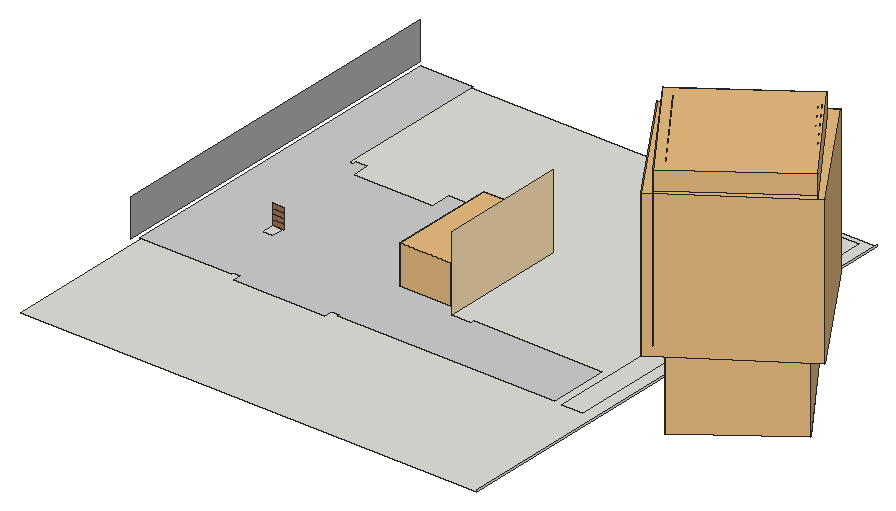
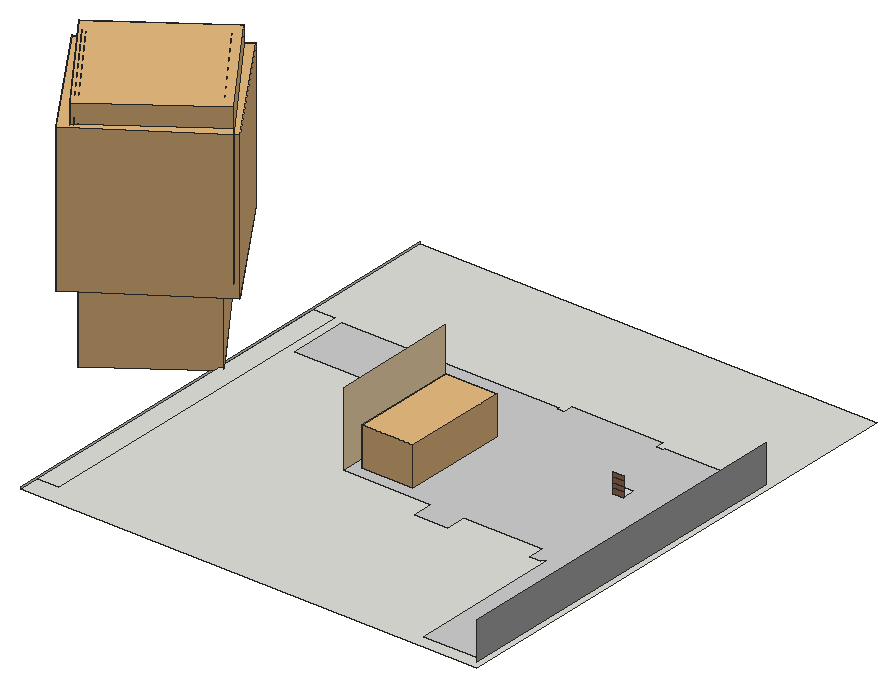
# SketchUp Ruby script. Lengths in inches.
U = 1.inch
M = Sketchup.active_model
def pt(a) = Geom::Point3d.new(a.map { |v| v * U })
def face(e, loops, mat)
  f = e.add_face(loops[0].map { |a| pt(a) })
  loops[1..].each { |l| e.add_face(l.map { |a| pt(a) }).erase! }
  f.material = f.back_material = mat if mat
  f
end
# faces: each face lists its corners as indices into pts; further lists are holes
def faces(e, pts, list, mat = nil) = list.each { |f| face(e, (f[0].is_a?(Array) ? f : [f]).map { |l| l.map { |i| pts[i] } }, mat) }
# xy, xz, yz: faces in a plane at the given z, y or x. An outline is a flat list of corners, or four numbers for a rectangle; further outlines are holes
def ring(l) = l.size == 4 ? [[l[0], l[1]], [l[2], l[1]], [l[2], l[3]], [l[0], l[3]]] : l.each_slice(2).to_a
def flat(e, list, mat, &to3) = list.each { |f| face(e, (f[0].is_a?(Array) ? f : [f]).map { |l| ring(l).map { |u, v| to3.(u, v) } }, mat) }
def xy(e, z, list, mat = nil) = flat(e, list, mat) { |x, y| [x, y, z] }
def xz(e, y, list, mat = nil) = flat(e, list, mat) { |x, z| [x, y, z] }
def yz(e, x, list, mat = nil) = flat(e, list, mat) { |y, z| [x, y, z] }
def lines(e, pts, list) = list.each { |a, b| e.add_line(pt(pts[a]), pt(pts[b])) }
# prism: a flat outline (further loops are holes) pulled along v
def prism(e, loops, v, mat = nil)
  f = face(e, loops, mat); d = Geom::Vector3d.new(v.map { |x| x * U })
  f.pushpull(f.normal.samedirection?(d) ? d.length : -d.length)
end
def box(e, o, s, mat = nil) = prism(e, [[o, [o[0] + s[0], o[1], o[2]], [o[0] + s[0], o[1] + s[1], o[2]], [o[0], o[1] + s[1], o[2]]]], [0, 0, s[2]], mat)
def at(x, y, z, deg = 0) = Geom::Transformation.translation(pt([x, y, z])) * Geom::Transformation.rotation(ORIGIN, Z_AXIS, deg.degrees)
def axes(o, x, y, z) = Geom::Transformation.new([*x, 0, *y, 0, *z, 0, *pt(o).to_a, 1])
def part(name) = M.definitions.add(name)
# library, detail: a bought-in or finely detailed component or shape, given as its bounding box
def library(name, o, s) = part(name).tap { |d| box(d.entities, o, s) }
def detail(e, o, s) = box(e.add_group.entities, o, s)
def put(e, d, t, mat = nil) = e.add_instance(d, t).tap { |i| i.material = mat if mat }
def group(e, t, mat = nil) = e.add_group.tap { |g| g.transformation = t; g.material = mat if mat }.entities
root = M.entities
M.materials.add("028_190k_fullGeometry_Material \#4").color = [120, 148, 64]
M.materials.add("Colorsadfasdfa0sd1f06w3").color = [153, 130, 61]
M.materials.add("Euphorbia asdfasd0f150160s159w").color = [180, 173, 131]
M.materials.add("Euphorbiaasdfa0sdf1a56sd016wow Leaf SU").color = [141, 134, 72]
M.materials.add("[0032_Moccasin]").color = [255, 228, 181]
M.materials.add("[0132_LightGray]").color = [169, 169, 169]
M.materials.add("[Carrera Marble]").color = [207, 207, 207]
M.materials.add("[Tile Ceramic Multi]").color = [165, 115, 84]
M.materials.add("asdfasdf0165f6asdLeafVar1sfd015as60f1as6").color = [231, 235, 211]
M.materials.add("dw_stemssadfasdfa0sdf1s01d6w1").color = [90, 97, 50]
M.materials.add("viburnumblaasdfas0df1w06d").color = [98, 102, 84]
M.materials.add("viburnumbladsadfasdfad0w122").color = [125, 129, 119]
c1 = part("Component\#315")
p = [[0.25,0,0],[2.05,0.01,0.35],[1.81,4.2,1.66],[0,4.19,1.3125]]
faces(c1.entities,p,[[0,1,2,3]],"viburnumbladsadfasdfad0w122")
c2 = part("viburnumblad2")
put(c2.entities,c1,axes([-19.23,-4.49,-32.18],[83.35428,0,0],[0,79.38502,0],[0,0,83.35428]))
c3 = part("Component\#314")
p = [[0.14,0,0],[2.58,0.05,0.25],[2.44,5.11,2.64],[0,5.05,2.39]]
faces(c3.entities,p,[[0,1,2,3]],"viburnumblaasdfas0df1w06d")
c4 = part("viburnumblad1\#2")
put(c4.entities,c3,axes([-37.25,6.23,19.31],[75.98784,0,0],[0,65.50676,0],[0,0,75.98784]))
c5 = library("Narrowleaf plant",[-0.44,-0.75,-1.28],[7.48,8.05,9.01])
c6 = part("vdw_leaf\#3")
p = [[0,0,0],[-2.77,1.61,2.32],[-4.3125,6.1,4.5],[-3.97,13.49,6.09],[-2.47,18.57,6.3],[-0.2,22.73,5.75],
  [2.54,19.66,6.85],[4.3,15.93,7.09],[5.03,7.6,5.43],[3.32,1.76,2.74]]
faces(c6.entities,p,[[0,1,2,3,4,5],[0,5,6,7,8,9]],"asdfasdf0165f6asdLeafVar1sfd015as60f1as6")
c7 = part("dw_brancj_2\#2")
p = [[9.7,-0.22,29.95],[0.23,-1.96,0.34],[-0.05,1.51,0.11],[9.65,1.51,29.46],[18.64,-8.75,84.43],[18.96,-6.63,84.625],
  [1.53,6.02,63.68],[1.42,8.18,63.25],[-10.58,8.77,161.17],[-10.41,9.98,160.68],[26.34,-9.37,211.72],[26.57,-8.28,211.23]]
faces(c7.entities,p,[[0,1,2],[0,2,3],[4,0,3],[4,3,5],[6,0,3],[6,3,7],[8,6,7],[8,7,9],
  [10,4,5],[10,5,11]],"dw_stemssadfasdfa0sdf1s01d6w1")
c8 = part("vdw_branch2\#3")
put(c8.entities,c6,axes([19.53,-5.9,102.42],[1.12377,-0.50004,0],[0.46097,1.03596,0.47664],[-0.19377,-0.43548,1.13389]))
put(c8.entities,c6,axes([-5.89,6.52,109.44],[-1.07209,0.83679,0],[-0.77141,-0.98832,0.52702],[0.32427,0.41545,1.25373]))
put(c8.entities,c6,axes([-0.44,8.23,75.28],[0.88709,-0.9947,0],[0.92159,0.82189,0.33087],[-0.25219,-0.22491,1.26111]))
put(c8.entities,c6,axes([24.71,-8.97,190.81],[-0.82641,0.91101,0],[-0.83983,-0.76184,0.47664],[0.35303,0.32025,1.13389]))
put(c8.entities,c6,axes([-2.29,8.24,91.35],[1.24603,-0.47303,0],[0.43826,1.15445,0.33087],[-0.11993,-0.31592,1.26111]))
put(c8.entities,c6,axes([12.26,-3.11,37.92],[-0.64625,1.02205,0.22511],[-1.04383,-0.61044,-0.22511],[-0.07533,-0.30931,1.18809]))
put(c8.entities,c6,axes([26.17,-9.17,210.27],[-0.99452,-0.10453,0],[0.09636,-0.91681,0.38752],[-0.04051,0.38539,0.92186]))
put(c8.entities,c6,axes([-6.07,9.4,125.35],[-0.90214,-0.98107,0],[0.90896,-0.83583,0.33087],[-0.24874,0.22873,1.26111]))
put(c8.entities,c6,axes([-4.13,7.29,110.58],[0.44715,-1.078,0.64369],[1.05816,0.63649,0.33087],[-0.58725,0.40856,1.09216]))
put(c8.entities,c6,axes([23.91,-8.22,171.96],[0.62307,0.85009,-0.63406],[-0.71531,0.8798,0.47664],[0.78296,0.12729,0.94004]))
put(c8.entities,c7,at(-0.09,0.18,-0.25),"dw_stemssadfasdfa0sdf1s01d6w1")
put(c8.entities,c6,axes([23.34,-9.65,156.59],[-0.31364,-1.00782,0.58216],[1.10369,-0.17062,0.29925],[-0.17137,0.6239,0.98776]))
put(c8.entities,c6,axes([15.03,-3.37,58.83],[-1.05425,-0.00194,0.58442],[-0.14303,-1.11707,-0.26172],[0.55355,-0.3046,0.99755]))
put(c8.entities,c6,axes([-11.625,9.46,160.37],[0.36812,0.92978,0],[-0.85713,0.33936,0.38752],[0.3603,-0.14265,0.92186]))
put(c8.entities,c6,axes([21.32,-8.53,138.72],[1.21379,0.19904,0],[-0.19904,1.21379,0],[0,0,1.23]))
put(c8.entities,c6,axes([22.54,-9.2,141.43],[-1.02887,0.17955,0.60182],[-0.23387,-1.13057,-0.06253],[0.56696,-0.17376,1.02111]))
put(c8.entities,c6,axes([23.9,-8.82,173.84],[-1.14567,-0.37474,0],[0.35918,-1.0981,0.04438],[-0.01409,0.04308,1.17993]))
put(c8.entities,c6,axes([-7.84,8.92,143.59],[-1.26971,0.40522,0],[-0.37543,-1.17638,0.33087],[0.10274,0.32192,1.26111]))
put(c8.entities,c6,axes([19.77,-8.01,85.98],[-0.32405,-1.14591,0.18674],[1.10278,-0.32969,-0.10948],[0.15845,0.14442,1.16117]))
put(c8.entities,c6,axes([-0.62,5.76,76.34],[-0.08879,1.17576,-0.67771],[-1.34525,-0.16582,-0.11144],[-0.17897,0.66309,1.17383]))
put(c8.entities,c6,axes([20.49,-8.22,121.07],[0.39924,-0.78471,-0.8233],[1.08735,0.33121,0.2116],[0.09035,-0.83005,0.83495]))
put(c8.entities,c6,axes([15.15,-3.72,62.9],[1.16251,0.40128,-0.0211],[-0.39924,1.16074,0.07874],[0.0456,-0.06757,1.2273]))
put(c8.entities,c6,axes([20.72,-8.08,120.26],[-0.03693,1.2277,-0.06551],[-1.22944,-0.03698,0],[-0.00197,0.06548,1.22825]))
put(c8.entities,c6,axes([22.58,-8.36,155.57],[-0.56247,1.09386,0],[-1.00839,-0.51852,0.47664],[0.42389,0.21796,1.13389]))
put(c8.entities,c6,axes([3.97,3.13,57.96],[-1.09459,0.76041,0],[-0.72262,-1.0402,-0.1735],[-0.10109,-0.14552,1.29352]))
put(c8.entities,c6,axes([-10.8,9.06,160.75],[-0.66334,-0.72138,0],[0.66835,-0.61458,0.24329],[-0.1829,0.16818,0.92729]))
put(c8.entities,c6,axes([19.06,-9.3125,103.96],[-1.01345,0.25553,-0.60051],[-0.2265,-1.12952,-0.09839],[-0.59598,0.03076,1.01889]))
put(c8.entities,c6,axes([18.07,-6.2,81.7],[-0.56247,1.09386,0],[-1.00839,-0.51852,0.47664],[0.42389,0.21796,1.13389]))
put(c8.entities,c6,axes([12.95,-0.39,43.31],[0.13044,-1.19832,0],[1.11025,0.12085,0.29925],[-0.30382,-0.03307,1.14057]))
put(c8.entities,c6,axes([2.28,8.28,56.18],[1.32413,-0.31027,0],[0.30923,1.31968,-0.11144],[0.02542,0.1085,1.35543]))
put(c8.entities,c6,axes([-7.55,9.96,143.07],[1.34251,-0.21744,0],[0.20045,1.23761,0.52702],[-0.08426,-0.52024,1.25373]))
put(c8.entities,c6,axes([26.15,-8.25,210.66],[0.94661,-0.25364,0],[0.235,0.87703,0.24329],[-0.06431,-0.24,0.92729]))
put(c8.entities,c6,axes([-6.48,11.37,125.16],[0.64635,1.10315,0.46356],[-1.16569,0.46153,0.52702],[0.27017,-0.6478,1.16488]))
put(c8.entities,c6,axes([25.74,-8.35,191.28],[0.13044,-1.19832,0],[1.11025,0.12085,0.29925],[-0.30382,-0.03307,1.14057]))
put(c8.entities,c6,axes([-5.125,7.47,91.6],[-1.10024,0.63688,0.48318],[-0.78682,-1.00808,-0.46292],[0.14137,-0.65404,1.184]))
c9 = part("vdw_leaf\#2")
p = [[0,0,0],[-2.77,1.61,2.32],[-4.3125,6.1,4.5],[-3.97,13.49,6.09],[-2.47,18.57,6.3],[-0.2,22.73,5.75],
  [2.54,19.66,6.85],[4.3,15.93,7.09],[5.03,7.6,5.43],[3.32,1.76,2.74]]
faces(c9.entities,p,[[0,1,2,3,4,5],[0,5,6,7,8,9]],"asdfasdf0165f6asdLeafVar1sfd015as60f1as6")
c10 = part("dg_branch_1\#2")
p = [[46.12,1.57,35.62],[46,5.42,35.41],[0.14,1.79,0.05],[0.26,-2.0625,0.27],[74.05,2.99,75.8],[74.11,5.28,75.58],
  [103.46,0.47,94.74],[104.03,2.92,94.84],[81.14,16.92,120.46],[81.2,18.78,120.24],[130.47,-5.6875,130.27],[130.58,-3.66,129.85],
  [80.82,34.4375,191.22],[80.64,35.93,190.9],[148.49,-14.56,203.24],[148.9,-12.8125,203.11],[81.08,37.95,226.93],[81.4,39.1,227.03],
  [157.45,-18.19,250.77],[157.7,-17.01,250.41]]
faces(c10.entities,p,[[0,1,2,3],[4,0,1],[4,1,5],[6,4,5],[6,5,7],[8,4,5],[8,5,9],[10,6,7],
  [10,7,11],[12,8,9],[12,9,13],[14,10,11],[14,11,15],[16,12,13],[16,13,17],[18,14,15],
  [18,15,19]],"dw_stemssadfasdfa0sdf1s01d6w1")
c11 = part("vdw_branch1\#3")
put(c11.entities,c9,axes([120.69,-2.42,117.31],[1.12221,-0.24063,-0.65809],[0.19207,1.24776,-0.12871],[0.65778,0.01392,1.11658]))
put(c11.entities,c9,axes([81,38.9,226.05],[0.7888,-0.58155,0],[0.48308,0.65523,0.47],[-0.28484,-0.38635,0.83138]))
put(c11.entities,c9,axes([78.08,12.69,106.05],[-1.43826,-0.02353,-0.03177],[0.0088,-1.31777,0.57755],[-0.03854,0.57714,1.31741]))
put(c11.entities,c9,axes([130.18,-4.73,130.41],[-0.38031,-1.29044,-0.11242],[1.20662,-0.31032,-0.51987],[0.47109,-0.24694,1.24081]))
put(c11.entities,c9,axes([157.08,-17.89,249.93],[-0.91355,0.40674,0],[-0.37496,-0.84216,0.38752],[0.15762,0.35401,0.92186]))
put(c11.entities,c9,axes([90.64,3.03,86.49],[0.32514,-0.85045,-0.99675],[0.69523,0.98247,-0.61148],[1.11061,-0.36604,0.67459]))
put(c11.entities,c9,axes([80.15,28.42,160.95],[-0.16039,0.95636,-1.06292],[-1.41646,0.03966,0.24943],[0.19509,1.07422,0.93709]))
put(c11.entities,c9,axes([126.74,-5.45,129.22],[-0.59819,0.96152,-0.6841],[-0.85772,0.12575,0.92675],[0.75427,0.88089,0.57856]))
put(c11.entities,c9,axes([133.22,-6.12,150.66],[-0.93823,0.76985,0.59124],[-0.47726,-1.08188,0.65135],[0.84525,0.24366,1.02405]))
put(c11.entities,c9,axes([80.43,22.89,141.32],[-1.42571,-0.19312,0.01373],[0.18338,-1.31425,0.5561],[-0.0621,0.5528,1.32692]))
put(c11.entities,c9,axes([33.14,0.88,26.42],[-0.13338,1.31536,0.04876],[-1.04528,-0.13221,0.7073],[0.72315,0.03348,1.07497]))
put(c11.entities,c9,axes([152.63,-15.08,221.76],[-1.28188,0.41945,0.0579],[-0.3638,-1.18547,0.53367],[0.21665,0.49113,1.23869]))
put(c11.entities,c9,axes([80.05,28.28,160.33],[-0.46732,-1.26661,0.40679],[1.27397,-0.40257,0.21004],[-0.07408,0.44645,1.30501]))
put(c11.entities,c9,axes([153.95,-14.8,235.875],[0.39005,1.07743,0.20605],[-0.96443,0.25296,0.50293],[0.42961,-0.3464,0.99807]))
put(c11.entities,c9,axes([80.2,24.22,141.74],[1.33062,-0.46576,0.02628],[0.44746,1.2746,-0.06608],[-0.00197,0.0722,1.37936]))
put(c11.entities,c9,axes([145.48,-12.5,188.92],[-1.32952,0.16983,0.16138],[-0.09299,-1.2361,0.53471],[0.21503,0.51548,1.22904]))
put(c11.entities,c9,axes([139.64,-9.18,171.24],[0.05682,1.30088,0.23414],[-1.13176,-0.05343,0.57151],[0.58357,-0.22963,1.13417]))
put(c11.entities,c9,axes([70.95,4.35,71.98],[-1.1081,-0.41873,0.64752],[0.33675,-1.28259,-0.25313],[0.6937,-0.04625,1.15721]))
put(c11.entities,c9,axes([59.85,4.55,56.17],[-0.26797,1.24526,0.35754],[-0.9369,-0.41634,0.74783],[0.83377,-0.10389,0.98674]))
put(c11.entities,c9,axes([33.11,3.36,25.66],[-0.57817,-1.07968,-0.5679],[1.11554,-0.21356,-0.7297],[0.49375,-0.78178,0.98363]))
put(c11.entities,c10,at(-0.21,0.34,-0.17),"dw_stemssadfasdfa0sdf1s01d6w1")
put(c11.entities,c9,axes([80.91,19.01,122.53],[-0.84258,1.13222,-0.27981],[-1.15093,-0.75138,0.42537],[0.18861,0.47293,1.3457]))
put(c11.entities,c9,axes([119.8,-1.22,114.1],[-1.3235,-0.25012,0.09101],[0.25933,-1.31572,0.15537],[0.05991,0.1698,1.33794]))
put(c11.entities,c9,axes([46.29,5.1,38.04],[0.98937,0.73827,-0.47585],[-0.72359,1.03721,0.10473],[0.44068,0.18581,1.20453]))
put(c11.entities,c9,axes([81.1875,33.03,184.45],[1.33883,0.26986,0.35053],[-0.09581,1.22087,-0.57399],[-0.42216,0.53228,1.20262]))
put(c11.entities,c9,axes([80.16,36.28,206.98],[-0.83993,0.85737,-0.6234],[-1.05964,-0.65701,0.5241],[0.02941,0.81391,1.07976]))
put(c11.entities,c9,axes([154.86,-16.15,234.87],[0.02509,-1.15302,-0.28506],[1.1487,-0.04894,0.29908],[-0.30202,-0.28195,1.11384]))
put(c11.entities,c9,axes([108.77,-0.33,101.14],[-0.47691,-1.03266,-0.72709],[1.25395,-0.29455,-0.40416],[0.15052,-0.81814,1.06325]))
put(c11.entities,c9,axes([89.79,3.01,85.87],[-0.61344,0.75518,0.8965],[-0.17758,-1.01824,0.73622],[1.13385,0.22574,0.58569]))
put(c11.entities,c9,axes([81.56,20.31,123.29],[0.37259,-1.3435,0.21057],[1.29385,0.32364,-0.22445],[0.16906,0.25791,1.34638]))
put(c11.entities,c9,axes([46.45,1.82,36.74],[-0.77883,0.29892,1.0614],[0.19124,-1.24314,0.49044],[1.08598,0.43329,0.67484]))
put(c11.entities,c9,axes([71.37,4.02,72.32],[0.72905,0.81546,-0.74421],[-0.66805,0.98958,0.42988],[0.8391,0.14186,0.97745]))
put(c11.entities,c9,axes([136.59,-5.88,150.53],[0.85845,-0.99897,-0.12437],[0.96526,0.81273,0.13453],[-0.02572,-0.18182,1.28292]))
put(c11.entities,c9,axes([80.375,38.8,225.86],[-0.25178,0.96778,0],[-0.89216,-0.23211,0.38752],[0.37503,0.09757,0.92186]))
put(c11.entities,c9,axes([74.43,7.99,85.38],[-1.05703,0.91669,-0.33543],[-0.95806,-0.87958,0.61531],[0.18697,0.6754,1.25659]))
put(c11.entities,c9,axes([76.57,9.74,89.32],[0.63146,-1.21538,0.33508],[1.18148,0.49387,-0.43517],[0.26321,0.48577,1.26593]))
put(c11.entities,c9,axes([81.6875,36.97,207.4],[0.09422,-1.04424,0.38486],[1.01646,0.1939,0.27727],[-0.33299,0.33382,0.98727]))
put(c11.entities,c9,axes([157.29,-17.17,249.98],[0.50586,-0.50586,0],[0.38853,0.38853,0.41105],[-0.29684,-0.29684,0.56115]))
put(c11.entities,c9,axes([79.92,15.8,106.09],[1.03917,-0.29343,-0.90675],[-0.14587,1.22131,-0.5624],[0.92163,0.5191,0.88824]))
put(c11.entities,c9,axes([61.95,3.88,56.26],[0.41243,-1.28546,0],[1.17466,0.37688,-0.54831],[0.5221,0.16751,1.23363]))
put(c11.entities,c9,axes([151.99,-14.79,208.15],[-0.48571,-1.21723,-0.32393],[1.25386,-0.50033,0],[-0.12005,-0.30087,1.31056]))
put(c11.entities,c9,axes([108.44,0.62,102.22],[0.82183,0.96078,0.38967],[-0.62327,0.08618,1.10203],[0.79141,-0.88661,0.51693]))
put(c11.entities,c9,axes([145.6,-10.56,188.62],[1.03241,-0.02554,-0.82693],[0.3944,1.11584,0.45794],[0.70325,-0.61672,0.89706]))
put(c11.entities,c9,axes([78.59,32.3,183.89],[-1.12675,-0.42036,0.43987],[0.5899,-0.98149,0.57312],[0.14901,0.70693,1.05726]))
put(c11.entities,c9,axes([152.08,-13.42,223.37],[0.79993,-0.44251,-0.69938],[0.68456,0.82615,0.26026],[0.41048,-0.60953,0.85515]))
put(c11.entities,c9,axes([140.71,-8.74,170.55],[0.41903,-1.24177,-0.32393],[1.26224,0.33728,0.33986],[-0.23168,-0.40836,1.26573]))
put(c11.entities,c9,axes([149.25,-12.53,205.78],[1.24456,0.38285,0.23414],[-0.42999,1.04826,0.57151],[-0.02056,-0.62679,1.13417]))
c12 = part("Component\#306")
p = [[4.55,0.11,0],[4.55,0,0],[2.84,0,3.13],[2.84,0.11,3.13],[4.625,0.05,0.04],[2.92,0.05,3.15],
  [2.08,0,8.07],[2.08,0.11,8.07],[2.16,0.05,8.1],[0,0,12.54],[0,0.11,12.54],[0.07,0.05,12.58]]
faces(c12.entities,p,[[0,1,2,3],[1,4,5,2],[1,0,4],[4,0,3,5],[3,2,6,7],[2,5,8,6],[5,3,7,8],[7,6,9,10],
  [6,8,11,9],[8,7,10,11],[10,9,11]],"Colorsadfasdfa0sd1f06w3")
c13 = part("Component\#301")
xy(c13.entities,0,[[0,0,0.7,3.1]],"Euphorbiaasdfa0sdf1a56sd016wow Leaf SU")
c14 = part("Leaf rosette")
put(c14.entities,c13,axes([2.21,1.74,0.13],[-0.4441,0.47879,-0.0956],[-0.4878,-0.4406,0.05935],[-0.03146,0.16757,0.98536]))
put(c14.entities,c13,axes([2.29,1.9,0.17],[-0.62678,-0.10063,-0.18061],[0.01105,-0.59203,0.2915],[-0.31282,0.41486,0.85442]))
put(c14.entities,c13,axes([2.09,1.69,0.1],[-0.10438,0.65169,0],[-0.65169,-0.10438,0],[0,0,1]))
put(c14.entities,c13,axes([1.97,1.77,0.02],[0.31114,0.5228,0.25587],[-0.57125,0.32993,0.02052],[-0.16918,-0.3502,0.92127]))
put(c14.entities,c13,axes([1.93,1.95,0],[0.54816,-0.03215,0.36617],[-0.11878,0.60671,0.23108],[-0.52706,-0.39065,0.75472]))
put(c14.entities,c13,axes([2.04,2.1,0.05],[0.26275,-0.55867,0.23335],[0.34186,0.34684,0.44545],[-0.75711,-0.08556,0.64766]))
put(c14.entities,c13,axes([2.22,2.08,0.13],[-0.29265,-0.59104,-0.02512],[0.40323,-0.2198,0.47401],[-0.65583,0.2952,0.69479]))
c15 = part("Component\#308")
xy(c15.entities,0,[[0,0,5.01,4.64]],"Euphorbia asdfasd0f150160s159w")
c16 = part("Component\#316")
put(c16.entities,c12,at(2.35,3.5,0))
put(c16.entities,c14,at(0.25,1.59,12.45))
put(c16.entities,c15,axes([7.46,0.77,3.64],[0.10848,0.99337,0.03799],[-0.82378,0.11122,-0.55589],[-0.55643,0.02901,0.83038]))
put(c16.entities,c15,axes([1.97,2.58,1.93],[0.80762,-0.50565,0.30344],[0.47433,0.86274,0.17519],[-0.35038,0.00244,0.93661]))
put(c16.entities,c15,axes([5.79,0.14,3.9],[0.5013,0.78918,0.35482],[-0.74775,0.60146,-0.2813],[-0.4354,-0.1243,0.89162]))
put(c16.entities,c15,axes([1.87,2.6,3.75],[0.73154,-0.49698,0.46676],[0.47433,0.86274,0.17519],[-0.48976,0.09324,0.86686]))
put(c16.entities,c15,axes([3.91,7.06,6.66],[-0.50827,-0.83837,-0.19699],[0.8278,-0.53869,0.15675],[-0.23753,-0.08339,0.96779]))
put(c16.entities,c15,axes([1.2,3.99,6.83],[0.56066,-0.79708,0.22433],[0.74237,0.60386,0.29025],[-0.36682,0.0038,0.93028]))
put(c16.entities,c13,axes([2.42,3.73,12.57],[-0.1322,-0.64472,0.04955],[0.10064,0.02944,0.65162],[-0.9678,0.2092,0.14002]))
put(c16.entities,c13,axes([2.57,3.43,12.63],[-0.62833,0.089,-0.18134],[-0.19954,-0.36568,0.51192],[-0.04764,0.82148,0.56824]))
put(c16.entities,c15,axes([4.04,6.92,11.09],[-0.67411,-0.5063,-0.5378],[0.44628,-0.85937,0.24964],[-0.58857,-0.07172,0.80526]))
put(c16.entities,c13,axes([2.5,3.49,12.74],[-0.62833,0.089,-0.18134],[-0.18746,-0.03618,0.63178],[0.11402,0.98935,0.09049]))
put(c16.entities,c13,axes([2.3,3.27,12.51],[0.02916,0.64747,0.12464],[-0.56235,-0.04072,0.34308],[0.5216,-0.18387,0.83314]))
put(c16.entities,c15,axes([0.26,4.96,9.69],[0.33661,-0.92735,0.16343],[0.73504,0.36725,0.56995],[-0.58857,-0.07172,0.80526]))
put(c16.entities,c15,axes([4.76,6.31,12.62],[-0.95056,-0.1129,-0.28929],[0.09021,-0.99179,0.09066],[-0.29715,0.06008,0.95294]))
put(c16.entities,c15,axes([5.2,6.55,10.37],[-0.76372,-0.27738,-0.58291],[0.26517,-0.95808,0.10848],[-0.58857,-0.07172,0.80526]))
c17 = part("Plant stem")
p = [[2.84,0.11,3.13],[2.84,0,3.13],[2.08,0,8.07],[2.08,0.11,8.07],[2.92,0.05,3.15],[2.16,0.05,8.1],
  [0,0,12.54],[0,0.11,12.54],[0.07,0.05,12.58]]
faces(c17.entities,p,[[0,1,2,3],[1,4,5,2],[4,0,3,5],[3,2,6,7],[2,5,8,6],[5,3,7,8],[7,6,8]],"Colorsadfasdfa0sd1f06w3")
c18 = part("Leafy shoot")
put(c18.entities,c17,at(2.35,3.5,0))
put(c18.entities,c14,at(0.25,1.59,12.45))
put(c18.entities,c15,axes([1.87,2.6,3.75],[0.73154,-0.49698,0.46676],[0.47433,0.86274,0.17519],[-0.48976,0.09324,0.86686]))
put(c18.entities,c15,axes([3.91,7.06,6.66],[-0.50827,-0.83837,-0.19699],[0.8278,-0.53869,0.15675],[-0.23753,-0.08339,0.96779]))
put(c18.entities,c15,axes([1.2,3.99,6.83],[0.56066,-0.79708,0.22433],[0.74237,0.60386,0.29025],[-0.36682,0.0038,0.93028]))
put(c18.entities,c13,axes([2.42,3.73,12.57],[-0.1322,-0.64472,0.04955],[0.10064,0.02944,0.65162],[-0.9678,0.2092,0.14002]))
put(c18.entities,c13,axes([2.57,3.43,12.63],[-0.62833,0.089,-0.18134],[-0.19954,-0.36568,0.51192],[-0.04764,0.82148,0.56824]))
put(c18.entities,c15,axes([4.04,6.92,11.09],[-0.67411,-0.5063,-0.5378],[0.44628,-0.85937,0.24964],[-0.58857,-0.07172,0.80526]))
put(c18.entities,c13,axes([2.5,3.49,12.74],[-0.62833,0.089,-0.18134],[-0.18746,-0.03618,0.63178],[0.11402,0.98935,0.09049]))
put(c18.entities,c13,axes([2.3,3.27,12.51],[0.02916,0.64747,0.12464],[-0.56235,-0.04072,0.34308],[0.5216,-0.18387,0.83314]))
put(c18.entities,c15,axes([0.26,4.96,9.69],[0.33661,-0.92735,0.16343],[0.73504,0.36725,0.56995],[-0.58857,-0.07172,0.80526]))
put(c18.entities,c15,axes([4.76,6.31,12.62],[-0.95056,-0.1129,-0.28929],[0.09021,-0.99179,0.09066],[-0.29715,0.06008,0.95294]))
put(c18.entities,c15,axes([5.2,6.55,10.37],[-0.76372,-0.27738,-0.58291],[0.26517,-0.95808,0.10848],[-0.58857,-0.07172,0.80526]))
put(c18.entities,c15,axes([7.03,0.77,3.77],[0.19714,0.84663,0.32426],[-0.94994,0.28899,-0.30484],[-0.2731,-0.45173,0.91532]))
c19 = part("Groundcover plant")
put(c19.entities,c16,axes([0.82,1.83,0.8125],[0.98541,0,-0.17021],[0,1,0],[0.17021,0,0.98541]))
put(c19.entities,c18,axes([4.45,-0.84,-2.24],[0.69527,0.50616,0],[-0.50264,0.69042,-0.10135],[-0.05965,0.08194,0.85401]))
put(c19.entities,c18,axes([1.85,7.37,-3.38],[0.7038,-0.47341,0.14191],[0.46407,0.71797,0.09357],[-0.16999,0,0.84303]))
put(c19.entities,c18,axes([6.9,-3.65,-2.52],[0.79351,0.57769,0],[-0.57366,0.78798,-0.11567],[-0.06808,0.09351,0.97468]))
put(c19.entities,c18,axes([1.36,5.18,-2.66],[0.50674,-0.34086,0.10218],[0.33413,0.51694,0.06737],[-0.12239,0,0.60698]))
put(c19.entities,c18,axes([5.76,-1.49,-2.17],[0.43479,0.43181,0.07251],[-0.43488,0.43544,-0.06951],[-0.06212,-0.06169,0.61918]))
c20 = part("Groundcover clump")
put(c20.entities,c19,axes([25.06,6.72,0.82],[-0.74291,1.22188,0],[-1.22188,-0.74291,0],[0,0,1]))
put(c20.entities,c19,axes([-0.76,2.1875,0.82],[1.43,0,0],[0,1.43,0],[0,0,1]))
put(c20.entities,c19,axes([8.21,24.79,0.82],[-0.6403,-1.27864,0],[1.27864,-0.6403,0],[0,0,1]))
c21 = library("028_190k_fullGeometry_0",[-319.99,-281.1,-2.15],[577.33,562.38,1159.36])
c22 = library("028_190k_fullGeometry_1",[-333.4,-281.7,421.48],[600.33,578.53,738.83])
c23 = library("028_190k_fullGeometry_2",[-3584003,-3264710,4041818.25],[6566285.5,6460741.75,7903602.75])
c24 = library("028_190k_fullGeometry_3",[-353.86,-324.57,405.22],[652.24,636.69,781.83])
c25 = part("028_190k_fullGeometry_4")
p = [[125.51,152.8,882.93],[125.36,152.82,883.01],[124.8,155.5625,881.05]]
faces(c25.entities,p,[[0,1,2]],"028_190k_fullGeometry_Material \#4")
c26 = part("028_190k_fullGeometry")
g1 = group(c26.entities,at(0,0,0))
put(g1,c21,axes([0,0,0],[0.18998,-0.26642,0],[0.26642,0.18998,0],[0,0,0.32722]))
put(g1,c22,axes([0,0,0],[0.18998,-0.26642,0],[0.26642,0.18998,0],[0,0,0.32722]))
put(g1,c23,axes([0,0,0],[0.00002,-0.00003,0],[0.00003,0.00002,0],[0,0,0.00003]))
put(g1,c24,axes([0,0,0],[0.18998,-0.26642,0],[0.26642,0.18998,0],[0,0,0.32722]))
put(g1,c25,axes([0,0,0],[0.18998,-0.26642,0],[0.26642,0.18998,0],[0,0,0.32722]))
c27 = library("Evoque+Azul+Marinho+As+Novinha+Fica+Loca+2017",[-10.19,-69.08,0],[168.96,82.02,63.04])
xy(root,-9,[[1338.625,0,2076.625,807.5]])
xy(root,0,[[2031.3125,228.9375,2065.5625,786.1875]])
xy(root,0,[[[1507.11,221.5,1654.31,221.5,1654.31,235.125,1666.62,235.125,1666.62,231.9375,2017.03,231.9375,2017.03,327.3125,1809.4375,327.3125,1809.4375,322.5,1777.8125,322.5,1777.8125,528.0625,1636.42,528.0625,1636.42,560.625,1583.17,560.625,1583.17,528.0625,1454.9375,528.0625,1454.9375,555,1437.22,555,1437.22,549.6875,1431.3125,549.6875,1431.3125,799.5,1346.625,799.5,1346.625,231.9375,1494.42,231.9375,1494.42,235.125,1507.11,235.125],[1457.08,340.22,1474.64,362.07]]],"[Carrera Marble]")
xz(root,362.07,[[1457.08,0,1474.64,8],[1457.08,8,1474.64,16],[1457.08,16,1474.64,24],[1457.08,24,1474.64,32]],"[Tile Ceramic Multi]")
yz(root,1338.625,[[223.9375,0,807.5,60]],"[0132_LightGray]")
yz(root,1777.8125,[[322.5,0,528.0625,120]],"[0032_Moccasin]")
yz(root,2076.625,[[0,-9,807.5,-6]])
put(root,c2,axes([2202.84,354.75,26.44],[-0.00947,-0.00564,0.00547],[0.00849,-0.00835,0.00609],[0.00092,0.00846,0.01032]))
put(root,c4,axes([2200.5,352.23,21.53],[0.00481,-0.00968,0.00992],[0.01607,0.00349,-0.00438],[0.00046,0.01061,0.01012]))
put(root,c2,axes([2196.2,354.17,26.83],[-0.01027,-0.00067,-0.00437],[-0.0029,-0.0054,0.00727],[-0.00275,0.0086,0.00434]))
put(root,c2,axes([2203.42,354.85,28.14],[-0.01295,0.00298,0.00152],[-0.00101,-0.00935,0.0097],[0.0032,0.00918,0.00919]))
put(root,c5,axes([2170.15,332.31,7.7],[0.15731,6.43674,0],[-6.43674,0.15731,0],[0,0,6.43866]))
put(root,c2,axes([2192.93,352.69,17.37],[0.00463,-0.00496,0.0092],[0.00608,0.00946,0.00204],[-0.0085,0.00407,0.00647]))
put(root,c2,axes([2195.15,353.72,27.01],[0.0028,0.00563,-0.00742],[-0.01015,0.00031,-0.00351],[-0.00158,0.00853,0.00492]))
put(root,c2,axes([2195.63,354.83,27.67],[-0.00494,0.0045,-0.00826],[-0.00853,-0.00405,0.00272],[-0.002,0.0084,0.00497]))
put(root,c2,axes([2203.13,352.58,23.875],[0.01322,0.00136,0.00142],[-0.00064,0.01212,-0.00561],[-0.00186,0.00548,0.01205]))
put(root,c2,axes([2195.68,354.78,25.74],[-0.00274,-0.00672,0.00719],[0.01014,0.00172,0.00518],[-0.00429,0.00766,0.00474]))
put(root,c2,axes([2195.87,355.66,26.76],[-0.00898,-0.00541,0.00233],[0.00475,-0.00369,0.00928],[-0.0037,0.00829,0.00425]))
put(root,c2,axes([2202.26,356.15,27.42],[-0.00139,-0.01031,0.00841],[0.01214,-0.00182,-0.00024],[0.00145,0.00829,0.0104]))
put(root,c2,axes([2195.61,356.22,28.08],[-0.00984,-0.00064,-0.00419],[-0.00322,-0.006,0.00808],[-0.00275,0.0086,0.00434]))
put(root,c2,axes([2201.45,355.14,26.41],[0.00854,-0.00981,0.00509],[0.00939,0.0055,-0.00515],[0.00179,0.0073,0.01107]))
put(root,c4,axes([2200.15,352.89,24.16],[0.01373,-0.0042,0.00303],[0.00601,0.01319,-0.00893],[-0.00014,0.00827,0.01212]))
put(root,c2,axes([2201.97,354.375,28.94],[0.00139,0.01031,-0.00841],[-0.01248,0.00393,0.00276],[0.0046,0.00756,0.01003]))
put(root,c2,axes([2201.13,353.84,27.46],[0.00973,0.00497,-0.00674],[-0.00836,0.01112,-0.00387],[0.00402,0.00678,0.0108]))
put(root,c8,axes([2172.49,352.66,6.3],[-0.13136,0.05263,-0.10053],[-0.06077,-0.15168,0],[-0.07584,0.03038,0.17413]))
put(root,c2,axes([2194.23,354.77,27.09],[0.00898,0.00541,-0.00233],[-0.00533,0.00547,-0.00762],[-0.00249,0.00719,0.00626]))
put(root,c8,axes([2177.12,350.94,5.4],[0.12089,0.06455,-0.10951],[-0.07696,0.14414,0],[0.0785,0.04192,0.16863]))
put(root,c2,axes([2194.38,355.64,28.19],[0.00286,0.007,-0.00749],[-0.01015,0.00031,-0.00351],[-0.0019,0.00782,0.00576]))
put(root,c4,axes([2205.24,354.69,16.8125],[0.00536,0.01158,-0.00521],[-0.01304,0.00197,-0.00903],[-0.0059,0.00728,0.01011]))
put(root,c2,axes([2194.78,355.67,26.22],[0.00494,-0.0045,0.00826],[0.00853,0.00632,-0.00167],[-0.00419,0.00708,0.00554]))
put(root,c2,axes([2204.91,357.27,18.93],[-0.00484,0.0048,-0.00995],[-0.01148,-0.00686,0.00228],[-0.0044,0.00962,0.00678]))
put(root,c2,axes([2195.18,356.89,27],[-0.00286,-0.007,0.00749],[0.00939,0.00159,0.0048],[-0.00429,0.00766,0.00474]))
put(root,c2,axes([2201.15,355.47,28.31],[0.01295,-0.00298,-0.00152],[0.00183,0.01176,-0.00745],[0.00286,0.00667,0.01124]))
put(root,c2,axes([2204.69,358.76,19.68],[-0.01065,-0.00175,-0.00643],[-0.00418,-0.00769,0.00902],[-0.00519,0.00978,0.00593]))
put(root,c2,axes([2201.94,357.16,29],[0.00818,-0.0094,0.00487],[0.01043,0.00611,-0.00572],[0.00179,0.0073,0.01107]))
put(root,c2,axes([2193.96,356.32,27.12],[0.00984,0.00064,0.00419],[0.00246,0.0079,-0.00679],[-0.00344,0.00689,0.00616]))
put(root,c2,axes([2201.49,355.94,30.08],[0.01014,0.00518,-0.00703],[-0.00774,0.0103,-0.00358],[0.00402,0.00678,0.0108]))
put(root,c2,axes([2203.53,357.95,19.7],[0.00352,0.00882,-0.00823],[-0.01182,-0.0007,-0.00581],[-0.00432,0.00892,0.00772]))
put(root,c2,axes([2203.37,359.19,20.93],[-0.00504,0.005,-0.01036],[-0.01063,-0.00635,0.00211],[-0.0044,0.00962,0.00678]))
put(root,c2,axes([2203.58,357.17,18.05],[0.01046,0.00781,-0.00132],[-0.00513,0.00543,-0.00849],[-0.00501,0.0081,0.0082]))
put(root,c2,axes([2204.04,360.33,20.04],[-0.01002,-0.00748,0.00127],[0.00432,-0.00389,0.01114],[-0.00624,0.00932,0.00567]))
put(root,c8,axes([2177.39,355.39,5.57],[-0.10999,0.0642,-0.09048],[-0.07413,-0.12701,0],[-0.0635,0.03707,0.15671]))
put(root,c2,axes([2202.85,358.46,18.49],[0.01065,0.00175,0.00643],[0.00257,0.00902,-0.00671],[-0.00605,0.00763,0.00794]))
put(root,c8,axes([2178.3125,356.05,8.3],[0.02088,0.1592,-0.03733],[-0.16201,0.02125,0],[0.00395,0.03008,0.19757]))
put(root,c2,axes([2202.12,359.17,19.95],[0.01002,0.00748,-0.00127],[-0.0057,0.00603,-0.00944],[-0.00501,0.0081,0.0082]))
put(root,c11,axes([2176.29,354.35,7.18],[-0.01089,0.12699,0],[-0.12699,-0.01089,0],[0,0,0.15683]))
put(root,c20,axes([2167.64,348.19,7.84],[1.49047,0,0],[0,1.49047,0],[0,0,1.49047]))
put(root,c26,at(2197.85,383.16,-5.3))
put(root,c27,at(1693.51,350.45,0,90))
